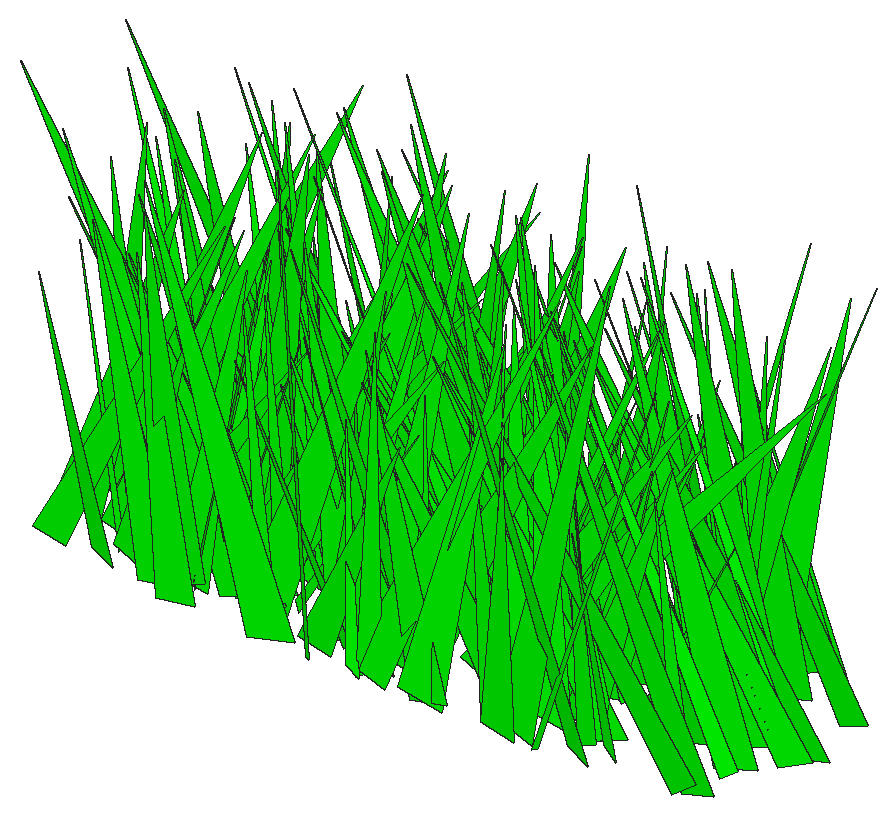
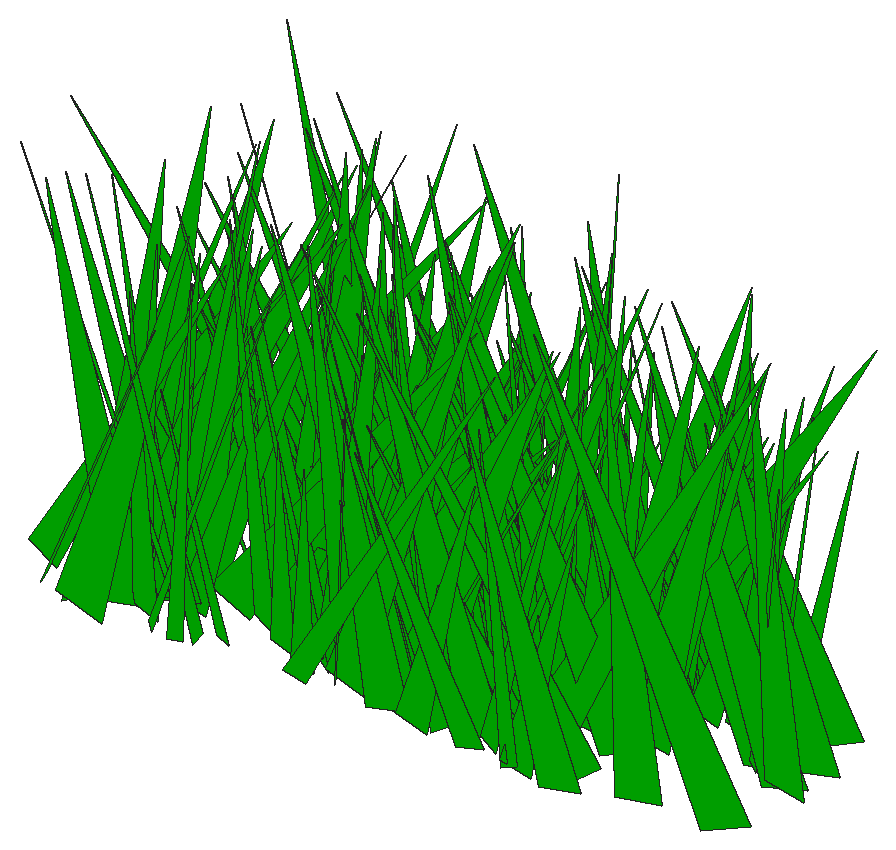
# SketchUp Ruby script. Lengths in inches.
U = 1.inch
M = Sketchup.active_model
def pt(a) = Geom::Point3d.new(a.map { |v| v * U })
def face(e, loops, mat)
  f = e.add_face(loops[0].map { |a| pt(a) })
  loops[1..].each { |l| e.add_face(l.map { |a| pt(a) }).erase! }
  f.material = f.back_material = mat if mat
  f
end
# faces: each face lists its corners as indices into pts; further lists are holes
def faces(e, pts, list, mat = nil) = list.each { |f| face(e, (f[0].is_a?(Array) ? f : [f]).map { |l| l.map { |i| pts[i] } }, mat) }
# xy, xz, yz: faces in a plane at the given z, y or x. An outline is a flat list of corners, or four numbers for a rectangle; further outlines are holes
def ring(l) = l.size == 4 ? [[l[0], l[1]], [l[2], l[1]], [l[2], l[3]], [l[0], l[3]]] : l.each_slice(2).to_a
def flat(e, list, mat, &to3) = list.each { |f| face(e, (f[0].is_a?(Array) ? f : [f]).map { |l| ring(l).map { |u, v| to3.(u, v) } }, mat) }
def xy(e, z, list, mat = nil) = flat(e, list, mat) { |x, y| [x, y, z] }
def xz(e, y, list, mat = nil) = flat(e, list, mat) { |x, z| [x, y, z] }
def yz(e, x, list, mat = nil) = flat(e, list, mat) { |y, z| [x, y, z] }
def lines(e, pts, list) = list.each { |a, b| e.add_line(pt(pts[a]), pt(pts[b])) }
# prism: a flat outline (further loops are holes) pulled along v
def prism(e, loops, v, mat = nil)
  f = face(e, loops, mat); d = Geom::Vector3d.new(v.map { |x| x * U })
  f.pushpull(f.normal.samedirection?(d) ? d.length : -d.length)
end
def box(e, o, s, mat = nil) = prism(e, [[o, [o[0] + s[0], o[1], o[2]], [o[0] + s[0], o[1] + s[1], o[2]], [o[0], o[1] + s[1], o[2]]]], [0, 0, s[2]], mat)
def at(x, y, z, deg = 0) = Geom::Transformation.translation(pt([x, y, z])) * Geom::Transformation.rotation(ORIGIN, Z_AXIS, deg.degrees)
def axes(o, x, y, z) = Geom::Transformation.new([*x, 0, *y, 0, *z, 0, *pt(o).to_a, 1])
def part(name) = M.definitions.add(name)
# library, detail: a bought-in or finely detailed component or shape, given as its bounding box
def library(name, o, s) = part(name).tap { |d| box(d.entities, o, s) }
def detail(e, o, s) = box(e.add_group.entities, o, s)
def put(e, d, t, mat = nil) = e.add_instance(d, t).tap { |i| i.material = mat if mat }
def group(e, t, mat = nil) = e.add_group.tap { |g| g.transformation = t; g.material = mat if mat }.entities
root = M.entities
M.materials.add("[0065_Lime]").color = [0, 255, 0]
c1 = part("fur_instance\#9")
p = [[0.8125,0,1.79],[0.67,-0.02,1.48],[0,-0.11,0],[0,0.11,0]]
faces(c1.entities,p,[[0,1,2,3]])
put(root,c1,axes([108.88,22.01,1.48],[4.75681,0.31747,1.98714],[-1.73779,0.74773,-1.25061],[-2.83772,0.07427,4.09688]),"[0065_Lime]")
put(root,c1,axes([107.32,22.59,1.48],[6.25624,-0.79402,0.40121],[5.39104,0.86446,1.70714],[-1.76366,-0.17423,6.64148]),"[0065_Lime]")
put(root,c1,axes([109.46,19.48,1.48],[-4.41361,-0.5637,0.07811],[3.85361,-0.60101,-1.27006],[1.11893,-0.15362,4.68226]),"[0065_Lime]")
put(root,c1,axes([109.5,20.23,1.48],[-5.51832,-0.04616,1.49049],[-0.04816,-0.8017,-0.94997],[1.86099,-0.15763,4.39513]),"[0065_Lime]")
put(root,c1,axes([107.19,21.34,1.48],[0.70179,-0.92138,2.00617],[6.79563,0.00491,-1.49729],[1.70207,0.36029,5.15083]),"[0065_Lime]")
put(root,c1,axes([109.98,20.83,1.48],[1.44553,0.98915,0.74754],[-6.89592,0.22695,-1.23991],[-1.68599,-0.08018,5.71232]),"[0065_Lime]")
put(root,c1,axes([110.23,20.91,1.48],[-6.41375,-0.00562,1.37592],[-0.3444,-0.90798,-1.18641],[1.65658,-0.21051,5.08044]),"[0065_Lime]")
put(root,c1,axes([111.48,20.82,1.48],[-6.87392,0.44824,1.7955],[-3.78696,-0.91218,-1.96188],[0.84068,-0.44398,5.8435]),"[0065_Lime]")
put(root,c1,axes([111.86,22.17,1.48],[-7.88942,0.4529,0.7145],[-3.09052,-1.10969,0.99166],[1.2683,0.11323,6.86094]),"[0065_Lime]")
put(root,c1,axes([114.3,20.58,1.48],[-2.0795,-1.15537,3.24941],[8.27079,0.00739,3.59006],[-3.89334,0.6328,5.89095]),"[0065_Lime]")
put(root,c1,axes([107.39,22.47,1.48],[5.1427,-0.91278,1.2703],[6.65541,0.67577,-1.556],[0.58303,0.33719,6.55712]),"[0065_Lime]")
put(root,c1,axes([111.92,22.77,1.48],[-1.07651,1.07847,0.62911],[-7.57075,-0.12668,-1.29461],[-1.47884,-0.13655,6.16966]),"[0065_Lime]")
put(root,c1,axes([111.49,19.3,1.48],[0.79576,0.87208,1.47847],[-6.2297,0.17243,-1.18969],[-1.73544,-0.2191,4.94855]),"[0065_Lime]")
put(root,c1,axes([107.26,25.14,1.48],[-2.18706,1.12852,2.58398],[-7.41501,-0.48145,2.89338],[4.42819,-0.24882,6.12118]),"[0065_Lime]")
put(root,c1,axes([113.59,20.85,1.48],[-5.58166,-0.54943,0.1697],[3.77911,-0.74255,1.68284],[-1.02475,0.25424,5.28174]),"[0065_Lime]")
put(root,c1,axes([107.625,19.53,1.48],[6.43557,-0.59106,0.78827],[4.3016,0.85789,-1.68113],[0.35835,0.31678,6.02355]),"[0065_Lime]")
put(root,c1,axes([114.28,23.85,1.48],[-6.00567,-0.99,0.85658],[6.98711,-0.78092,2.16878],[-1.38798,0.35246,7.21128]),"[0065_Lime]")
put(root,c1,axes([108.49,21.82,1.48],[8.65109,-0.17974,0.61801],[0.66489,1.03061,3.88566],[-1.3309,-0.65345,5.95838]),"[0065_Lime]")
put(root,c1,axes([109.99,25.4375,1.48],[-2.32113,-1.09259,0.4435],[7.51688,-0.33492,-1.61844],[2.06205,-0.00898,6.39898]),"[0065_Lime]")
put(root,c1,axes([108.86,20.88,1.48],[4.52414,0.72389,0.76271],[-5.23046,0.61658,0.9183],[0.24588,-0.2033,5.50075]),"[0065_Lime]")
put(root,c1,axes([112.42,20.94,1.48],[-6.35456,0.66956,0.55453],[-4.63808,-0.89415,1.01161],[1.28754,0.08357,6.38094]),"[0065_Lime]")
put(root,c1,axes([112.68,21.36,1.48],[4.49242,0.96826,0.54109],[-5.75128,0.58404,-3.42722],[-3.85307,0.25715,5.74652]),"[0065_Lime]")
put(root,c1,axes([109.91,19.96,1.48],[-2.07932,-0.66053,1.31721],[4.38724,-0.3598,-1.46364],[2.33894,0.08769,3.91639]),"[0065_Lime]")
put(root,c1,axes([108.47,21.99,1.48],[5.47429,0.98354,0.81524],[-7.02248,0.73547,1.46742],[0.82545,-0.26578,7.07742]),"[0065_Lime]")
put(root,c1,axes([112.79,23.15,1.48],[0.36017,-1.13824,1.08313],[8.05483,0.08514,1.22574],[-1.58371,0.17414,6.48052]),"[0065_Lime]")
put(root,c1,axes([113.59,20.08,1.48],[-0.45294,0.79492,1.39232],[-5.53302,0.02778,-1.72246],[-2.07798,-0.24725,4.28287]),"[0065_Lime]")
put(root,c1,axes([112.48,18.79,1.48],[1.21549,0.89008,0.72447],[-6.21056,0.19472,-1.12208],[-1.53157,-0.08319,5.12502]),"[0065_Lime]")
put(root,c1,axes([112.08,19.625,1.48],[4.98292,-0.96258,0.19503],[6.39598,0.66793,2.34476],[-2.46469,-0.21275,6.47907]),"[0065_Lime]")
put(root,c1,axes([114.55,20.11,1.48],[-2.22166,0.79723,0.80505],[-5.49656,-0.24901,-1.77319],[-1.71947,-0.23408,4.62809]),"[0065_Lime]")
put(root,c1,axes([114,22.82,1.48],[-2.51218,0.56119,0.72618],[-4.00317,-0.30645,-1.2272],[-0.84932,-0.21549,3.63629]),"[0065_Lime]")
put(root,c1,axes([114.17,20.66,1.48],[-2.35921,-1.01795,0.20784],[7.1664,-0.32186,0.99863],[-1.08993,0.08714,6.11622]),"[0065_Lime]")
put(root,c1,axes([111.86,21.4,1.48],[-5.14477,0.60785,0.71079],[-3.35714,-0.66147,2.87761],[2.86458,0.3165,4.64899]),"[0065_Lime]")
put(root,c1,axes([113.64,22.29,1.48],[-6.77708,0.59996,0.57809],[-3.92781,-0.93039,1.88959],[1.81862,0.22633,6.23535]),"[0065_Lime]")
put(root,c1,axes([111.94,23.04,1.48],[4.32561,0.38631,0.37978],[-2.5286,0.59443,-1.20585],[-1.17567,0.14285,3.9908]),"[0065_Lime]")
put(root,c1,axes([114.08,20.16,1.48],[-0.38061,-0.81633,1.21559],[5.84728,-0.00353,1.13197],[-1.3388,0.21667,4.59834]),"[0065_Lime]")
put(root,c1,axes([110.14,20.54,1.48],[3.92345,-0.53628,0.94206],[3.819,0.43935,-2.14273],[1.14972,0.37068,3.90264]),"[0065_Lime]")
put(root,c1,axes([113.64,26.11,1.48],[1.01933,-0.67584,0.27572],[4.63432,0.15077,1.0475],[-1.33061,0.00736,3.85949]),"[0065_Lime]")
put(root,c1,axes([112.12,19.8,1.48],[2.95244,-0.66107,2.58793],[5.66677,0.3764,-1.05566],[-0.37755,0.47991,4.39281]),"[0065_Lime]")
put(root,c1,axes([113.6,23.21,1.48],[6.49926,-0.57584,2.86664],[4.03045,1.03237,0.90299],[-3.60122,0.11618,6.18415]),"[0065_Lime]")
put(root,c1,axes([112.33,19.8125,1.48],[6.78722,0.16059,1.38807],[-0.6006,0.94692,-1.72789],[-1.96403,0.26539,5.32521]),"[0065_Lime]")
put(root,c1,axes([115.75,18.77,1.48],[-4.23697,0.9376,1.31798],[-6.84398,-0.55507,-1.32537],[-0.5542,-0.31336,6.29115]),"[0065_Lime]")
put(root,c1,axes([116.09,23.7,1.48],[-9.10693,-0.06064,1.00007],[0.17761,-1.26614,-1.5026],[1.29085,-0.25362,7.26219]),"[0065_Lime]")
put(root,c1,axes([115.02,25.53,1.48],[-5.8261,-0.37077,1.50453],[3.04674,-0.8087,1.12797],[1.04928,0.28945,5.07865]),"[0065_Lime]")
put(root,c1,axes([111.99,26.27,1.48],[1.22642,-0.90787,0.30312],[6.29841,0.15519,-1.28521],[1.48734,0.09141,5.19254]),"[0065_Lime]")
put(root,c1,axes([112.79,20.4,1.48],[5.14158,0.13277,0.67971],[-0.67571,0.70606,-1.23959],[-1.0651,0.19299,4.06757]),"[0065_Lime]")
put(root,c1,axes([112.34,21.03,1.48],[-2.53483,0.95653,2.95117],[-7.12293,-0.49622,1.34139],[2.96051,-0.3749,5.75419]),"[0065_Lime]")
put(root,c1,axes([112.46,22.05,1.48],[0.56511,0.56516,0.38968],[-3.7117,0.04505,1.37222],[1.62152,-0.09385,3.00523]),"[0065_Lime]")
put(root,c1,axes([113.23,21.25,1.48],[0.21192,-1.1921,1.83278],[8.70845,-0.01117,-0.90969],[1.10098,0.31781,6.84266]),"[0065_Lime]")
put(root,c1,axes([114.74,23.37,1.48],[-4.45858,-0.65966,0.8551],[4.54422,-0.6436,-0.96036],[1.5791,-0.01043,5.17802]),"[0065_Lime]")
put(root,c1,axes([114.6,20.02,1.48],[-5.51128,0.12231,2.48203],[-2.12772,-0.77996,-1.83809],[2.35399,-0.41864,4.14963]),"[0065_Lime]")
put(root,c1,axes([115.2,22.08,1.48],[-7.4027,0.42566,2.73576],[-3.72336,-1.0878,-0.99465],[2.57381,-0.3494,6.4296]),"[0065_Lime]")
put(root,c1,axes([113.82,26.14,1.48],[5.24176,0.29944,2.16883],[-3.01127,0.72897,1.44279],[-1.60707,-0.38923,4.3706]),"[0065_Lime]")
put(root,c1,axes([117.45,23.07,1.48],[-6.65793,-0.86672,0.90402],[6.2657,-0.91523,1.12903],[-0.14464,0.24903,7.29565]),"[0065_Lime]")
put(root,c1,axes([111.94,23.67,1.48],[-3.03044,1.05577,2.21873],[-6.67995,-0.55962,2.88653],[4.38979,-0.12274,5.9241]),"[0065_Lime]")
put(root,c1,axes([115.4375,22.41,1.48],[1.84297,1.05998,1.58754],[-7.62241,0.30371,-0.94025],[-1.61588,-0.2237,6.24601]),"[0065_Lime]")
put(root,c1,axes([114.8125,20.5,1.48],[5.76147,-0.43307,1.32614],[2.30483,0.80508,2.18459],[-2.61617,-0.24446,4.84511]),"[0065_Lime]")
put(root,c1,axes([118.36,24.63,1.48],[-8.66441,0.10283,0.01318],[-0.72259,-1.20595,0.97318],[0.11668,0.16733,7.00557]),"[0065_Lime]")
put(root,c1,axes([116.27,23.9,1.48],[1.54175,0.61801,1.12889],[-4.15611,0.27531,-1.29491],[-1.99901,-0.09575,3.56289]),"[0065_Lime]")
put(root,c1,axes([114.83,22.57,1.48],[-2.20909,0.81477,0.06052],[-5.52498,-0.29913,1.51072],[1.76097,0.0836,4.81576]),"[0065_Lime]")
put(root,c1,axes([117.61,19.7,1.48],[-4.71309,-0.23078,0.31888],[1.6872,-0.63733,1.04366],[-0.06575,0.18829,3.92334]),"[0065_Lime]")
put(root,c1,axes([114.79,23.65,1.48],[-6.53595,-0.6054,2.38454],[3.40148,-0.99622,-2.30654],[3.94784,-0.14393,5.9351]),"[0065_Lime]")
put(root,c1,axes([113.04,20.89,1.48],[3.67559,-0.76857,0.24402],[5.32315,0.48917,-1.42317],[1.29237,0.171,5.16789]),"[0065_Lime]")
put(root,c1,axes([118.3125,24.52,1.48],[-2.28678,1.15619,0.4981],[-8.03755,-0.29199,-1.70332],[-1.86378,-0.15937,6.73442]),"[0065_Lime]")
put(root,c1,axes([111.93,25.12,1.48],[7.61782,-0.42793,0.14657],[2.94088,1.01199,-2.12453],[0.81116,0.34978,6.32601]),"[0065_Lime]")
put(root,c1,axes([111.79,22.7,1.48],[5.17986,-0.77049,0.06287],[5.04502,0.6637,-2.45936],[2.14937,0.299,5.62112]),"[0065_Lime]")
put(root,c1,axes([116.96,20.71,1.48],[-0.18332,-0.59721,0.87484],[4.22584,0.0162,0.95637],[-1.16707,0.15245,3.32548]),"[0065_Lime]")
put(root,c1,axes([117.81,20.99,1.48],[-7.05017,0.06409,0.7695],[-0.25595,-0.97987,1.18316],[1.01855,0.19739,5.62357]),"[0065_Lime]")
put(root,c1,axes([114.29,24.84,1.48],[-1.69328,-1.27873,0.40691],[8.7177,-0.2481,-2.12324],[2.65778,-0.00089,7.22362]),"[0065_Lime]")
put(root,c1,axes([117.32,25.92,1.48],[0.67945,0.70964,1.24411],[-5.01954,0.15375,-1.12489],[-1.62727,-0.17795,3.98934]),"[0065_Lime]")
put(root,c1,axes([115.96,24.12,1.48],[3.20358,0.43841,0.0671],[-2.92117,0.42703,-1.21601],[-1.09889,0.1429,3.42813]),"[0065_Lime]")
put(root,c1,axes([116.34,21.95,1.48],[-4.33322,-0.2806,1.31295],[1.69913,-0.64693,-0.92263],[1.92507,-0.06061,3.76969]),"[0065_Lime]")
put(root,c1,axes([117.49,20,1.48],[1.80855,1.06223,0.18183],[-7.2575,0.25285,-1.73635],[-2.12693,0.04045,6.07937]),"[0065_Lime]")
put(root,c1,axes([114.125,21.95,1.48],[-0.07185,1.2934,0.07562],[-8.85908,-0.01326,2.03283],[2.49988,-0.00983,7.2061]),"[0065_Lime]")
put(root,c1,axes([117.12,18.61,1.48],[7.88751,0.15029,3.42144],[-0.47652,1.24861,-1.11101],[-4.31389,0.13687,6.37848]),"[0065_Lime]")
put(root,c1,axes([120.32,24.45,1.48],[-4.53183,1.05701,0.11134],[-7.24742,-0.60731,-1.98181],[-2.01934,-0.19252,6.86289]),"[0065_Lime]")
put(root,c1,axes([119.54,22.58,1.48],[-7.74639,-0.18987,0.54799],[1.44778,-1.07452,1.06543],[0.42849,0.19802,6.3068]),"[0065_Lime]")
put(root,c1,axes([120.15,22.93,1.48],[-7.37445,0.23979,0.33216],[-1.70896,-0.92533,-2.71939],[-0.39788,-0.46995,5.52389]),"[0065_Lime]")
put(root,c1,axes([119.01,20.19,1.48],[-2.08243,0.70172,0.46791],[-4.84715,-0.25712,-1.35203],[-1.33208,-0.1614,4.18826]),"[0065_Lime]")
put(root,c1,axes([114.24,24.77,1.48],[3.79805,0.57077,0.31827],[-3.85368,0.47697,1.76436],[1.34222,-0.24566,4.16509]),"[0065_Lime]")
put(root,c1,axes([113.89,20.45,1.48],[3.51071,0.78023,0.49381],[-5.25387,0.42706,2.10303],[1.89635,-0.26126,4.91232]),"[0065_Lime]")
put(root,c1,axes([114.44,20.07,1.48],[6.76565,-0.83708,2.01476],[6.4503,0.88762,-1.97384],[-0.12735,0.48692,7.06186]),"[0065_Lime]")
put(root,c1,axes([115.89,23.16,1.48],[-3.1916,-0.77323,2.59515],[5.69373,-0.5709,-1.06685],[2.83556,0.27603,5.0632]),"[0065_Lime]")
put(root,c1,axes([115.28,25.98,1.48],[2.3863,0.6485,0.60605],[-4.56285,0.29752,1.21908],[1.01725,-0.18676,4.04648]),"[0065_Lime]")
put(root,c1,axes([114.39,22.34,1.48],[5.26977,-0.54033,0.30957],[3.79475,0.70663,-1.41195],[0.72856,0.22776,5.11503]),"[0065_Lime]")
put(root,c1,axes([115.15,20.64,1.48],[4.78228,0.13087,0.01494],[-0.89815,0.64419,1.12549],[0.24722,-0.19132,3.79988]),"[0065_Lime]")
put(root,c1,axes([115.42,25.35,1.48],[0.23421,-1.08101,2.16362],[7.81278,-0.07509,-1.81665],[2.28442,0.36762,5.99115]),"[0065_Lime]")
put(root,c1,axes([120.08,25.29,1.48],[4.54453,0.80887,4.60833],[-6.54285,0.90426,-1.04944],[-4.73539,-0.47314,5.87259]),"[0065_Lime]")
put(root,c1,axes([118.91,21.45,1.48],[-4.66798,0.18091,0.42592],[-1.08616,-0.6357,1.17185],[0.8672,0.17761,3.7604]),"[0065_Lime]")
put(root,c1,axes([116.48,25.56,1.48],[-5.97897,-0.8659,1.63522],[4.93662,-0.85736,-3.27031],[4.20046,-0.22491,6.17104]),"[0065_Lime]")
put(root,c1,axes([116.89,24.8,1.48],[-0.93274,0.72478,1.44432],[-5.25377,-0.18747,0.90751],[1.46789,-0.21044,4.16585]),"[0065_Lime]")
put(root,c1,axes([116.77,20.32,1.48],[-5.33037,0.70186,1.45724],[-3.84774,-0.75694,2.9042],[3.65413,0.22677,5.18378]),"[0065_Lime]")
put(root,c1,axes([119.18,19.52,1.48],[-5.78186,-0.32004,0.6774],[2.09686,-0.81176,-1.00964],[1.21821,-0.12171,4.95292]),"[0065_Lime]")
put(root,c1,axes([116.67,20.41,1.48],[7.33665,-0.52864,0.50322],[3.29109,0.97329,2.51445],[-1.9248,-0.35083,6.21738]),"[0065_Lime]")
put(root,c1,axes([121.33,25.88,1.48],[-7.42153,0.39429,0.17707],[-2.78536,-1.01665,-1.38433],[-0.40322,-0.23434,6.30361]),"[0065_Lime]")
put(root,c1,axes([120.53,19.48,1.48],[-6.78605,-0.44371,1.28341],[3.51607,-0.8922,1.96457],[0.31266,0.40299,5.76251]),"[0065_Lime]")
put(root,c1,axes([118.51,18.78,1.48],[-4.45554,0.29398,0.76074],[-1.6058,-0.6055,1.61806],[1.63496,0.20645,3.66233]),"[0065_Lime]")
put(root,c1,axes([116.86,19.22,1.48],[0.87841,-0.73867,0.02479],[5.04663,0.11728,-1.21777],[1.47184,0.03873,4.16068]),"[0065_Lime]")
put(root,c1,axes([122.1875,22.21,1.48],[-3.38223,-0.67748,0.64954],[4.32175,-0.35094,2.62408],[-2.28146,0.33957,4.00785]),"[0065_Lime]")
put(root,c1,axes([119.83,23.92,1.48],[-5.47386,-0.14391,1.0743],[0.66616,-0.77074,-1.21387],[1.53278,-0.17896,4.36409]),"[0065_Lime]")
put(root,c1,axes([117.8,20.84,1.48],[6.55865,-0.63822,2.86701],[5.55432,0.89734,-1.7134],[-1.48379,0.538,6.25893]),"[0065_Lime]")
put(root,c1,axes([120.92,22.9,1.48],[-3.03016,-1.18286,2.10117],[8.78455,-0.37977,1.2181],[-0.60401,0.41089,7.17464]),"[0065_Lime]")
put(root,c1,axes([121.56,22.23,1.48],[-0.58168,1.07553,3.09864],[-8.21284,0.07882,-1.93679],[-2.37608,-0.53573,5.93589]),"[0065_Lime]")
put(root,c1,axes([118.27,25.61,1.48],[5.00089,-0.23631,0.58981],[1.43452,0.68964,1.21137],[-1.13849,-0.16906,4.11713]),"[0065_Lime]")
put(root,c1,axes([118.9,19,1.48],[6.15038,-0.52199,1.19737],[3.22978,0.87297,1.77594],[-2.35269,-0.16618,5.56817]),"[0065_Lime]")
put(root,c1,axes([119.15,21.14,1.48],[5.05279,-0.24169,1.22034],[1.01446,0.69657,1.84367],[-2.04453,-0.25168,3.9307]),"[0065_Lime]")
put(root,c1,axes([121.82,21.36,1.48],[-5.27601,0.45464,0.36816],[-3.25893,-0.72395,-0.94344],[-0.22895,-0.17197,4.94507]),"[0065_Lime]")
put(root,c1,axes([117.53,25.19,1.48],[7.65657,0.04562,1.09105],[-0.73546,1.03397,1.96609],[-1.16776,-0.35207,5.91538]),"[0065_Lime]")
put(root,c1,axes([118.28,25.73,1.48],[-0.86023,-0.99421,0.49878],[6.80499,-0.14022,-1.60067],[2.0318,0.04871,5.57219]),"[0065_Lime]")
put(root,c1,axes([121.11,18.75,1.48],[1.35591,0.83981,1.29808],[-5.86256,0.24771,-1.31835],[-1.97382,-0.15883,4.80744]),"[0065_Lime]")
put(root,c1,axes([123.15,22.43,1.48],[-1.84543,-1.23425,1.90817],[8.65227,-0.13516,2.60709],[-2.79147,0.39704,6.81928]),"[0065_Lime]")
put(root,c1,axes([120.51,25.13,1.48],[-5.85625,0.07812,1.72253],[0.41265,-0.79512,2.13666],[2.15018,0.36538,4.28143]),"[0065_Lime]")
put(root,c1,axes([123.71,21.6,1.48],[-4.77751,0.58364,0.27694],[-3.75387,-0.57107,-2.5182],[-1.81001,-0.35615,4.49164]),"[0065_Lime]")
put(root,c1,axes([120.8125,24.79,1.48],[5.51324,-0.87776,0.99225],[5.64963,0.77936,2.33265],[-2.93089,-0.14883,6.36296]),"[0065_Lime]")
put(root,c1,axes([119.12,23.35,1.48],[0.62244,0.70849,0.87955],[-5.00092,0.04561,1.11055],[1.25776,-0.16928,3.98036]),"[0065_Lime]")
put(root,c1,axes([120.24,24.79,1.48],[6.49909,0.95529,0.52041],[-6.29431,0.88622,-2.50314],[-2.64731,0.23809,7.22911]),"[0065_Lime]")
put(root,c1,axes([121.32,22.29,1.48],[1.02109,-1.08574,0.0472],[7.64617,0.14316,0.90803],[-1.11425,-0.01255,6.27429]),"[0065_Lime]")
put(root,c1,axes([120.9375,23.125,1.48],[2.50794,0.80047,0.27755],[-5.56145,0.35456,-1.01625],[-1.27987,0.02786,4.95983]),"[0065_Lime]")
put(root,c1,axes([120.93,21.49,1.48],[-6.29754,0.28767,1.72302],[-0.88384,-0.85463,2.64386],[2.81013,0.37586,4.69286]),"[0065_Lime]")
put(root,c1,axes([123.21,19.71,1.48],[0.92262,-0.87538,0.67989],[5.52158,0.1696,2.35948],[-3.00327,0.04289,4.54682]),"[0065_Lime]")
put(root,c1,axes([118.5,24.87,1.48],[1.78241,-1.15471,0.51368],[8.00538,0.22097,-1.73401],[1.9597,0.14756,6.61622]),"[0065_Lime]")
put(root,c1,axes([117.92,21.88,1.48],[5.81279,0.63106,0.00545],[-4.41707,0.80308,1.08633],[0.8113,-0.14907,5.87539]),"[0065_Lime]")
put(root,c1,axes([120.27,21.86,1.48],[-4.69664,-0.91781,1.37829],[6.05408,-0.70126,-1.99813],[2.98014,-0.02186,6.2313]),"[0065_Lime]")
put(root,c1,axes([121.29,25.59,1.48],[-2.93693,0.50067,0.15322],[-3.41179,-0.40411,0.9779],[1.04414,0.08782,3.62633]),"[0065_Lime]")
put(root,c1,axes([125.1875,23.78,1.48],[-5.44815,0.81973,0.96618],[-5.55931,-0.61958,-3.1268],[-2.12979,-0.47965,5.69021]),"[0065_Lime]")
put(root,c1,axes([118.2,21.76,1.48],[7.16849,0.77844,1.90301],[-6.01271,0.91912,2.38724],[0.10214,-0.5272,6.97184]),"[0065_Lime]")
put(root,c1,axes([122.95,22.78,1.48],[-1.41699,0.72489,0.97846],[-5.13613,-0.14521,-1.3164],[-1.29585,-0.21709,4.14767]),"[0065_Lime]")
put(root,c1,axes([125.2,22.29,1.48],[-5.42074,0.38654,0.03939],[-2.52569,-0.69319,-2.03181],[-1.09104,-0.31582,4.50782]),"[0065_Lime]")
put(root,c1,axes([118.91,18.86,1.48],[6.33349,0.90822,0.60373],[-6.47232,0.86483,1.329],[0.65996,-0.23449,7.23979]),"[0065_Lime]")
put(root,c1,axes([120.85,18.72,1.48],[-2.78902,0.94375,1.61298],[-6.48391,-0.46132,1.6268],[2.64564,-0.1357,5.68732]),"[0065_Lime]")
put(root,c1,axes([121.3,24.77,1.48],[5.85912,0.47031,0.62649],[-3.00871,0.80608,-1.65999],[-1.65629,0.19945,5.23164]),"[0065_Lime]")
put(root,c1,axes([122.55,24.83,1.48],[2.14179,0.565,0.18937],[-3.86834,0.29889,-0.93463],[-1.12136,0.04807,3.58588]),"[0065_Lime]")
put(root,c1,axes([122.97,19.17,1.48],[3.0262,0.58862,1.21834],[-3.98394,0.47185,-1.09153],[-1.97955,-0.04979,4.05926]),"[0065_Lime]")
put(root,c1,axes([123.125,20.11,1.48],[-4.86138,0.82668,0.80414],[-5.69414,-0.69645,1.21537],[1.77897,0.02984,6.08763]),"[0065_Lime]")
put(root,c1,axes([122.45,21.97,1.48],[-3.25218,0.61462,0.68324],[-4.03718,-0.46852,1.4083],[1.88101,0.05706,4.2039]),"[0065_Lime]")
put(root,c1,axes([119.74,19.71,1.48],[4.44404,-0.97779,0.88545],[6.88012,0.564,-1.97731],[1.5065,0.30865,6.41829]),"[0065_Lime]")
put(root,c1,axes([124.98,23.11,1.48],[-0.84639,-0.78047,0.35779],[5.25673,-0.09114,1.56576],[-1.84652,0.09828,4.29344]),"[0065_Lime]")
put(root,c1,axes([126.1875,20.18,1.48],[-4.81737,0.65495,0.08588],[-4.48491,-0.64519,-1.57446],[-1.27345,-0.20537,5.22014]),"[0065_Lime]")
put(root,c1,axes([124.21,21.76,1.48],[2.5245,-1.16462,2.00194],[8.34624,0.42229,1.26832],[-2.25603,0.25906,6.93236]),"[0065_Lime]")
put(root,c1,axes([124.59,21.47,1.48],[-0.53859,-0.67612,1.08932],[4.83092,-0.02248,1.11288],[-1.26782,0.20158,3.77777]),"[0065_Lime]")
put(root,c1,axes([123.32,18.78,1.48],[5.75086,-0.0612,2.22428],[1.02934,0.8695,-0.95913],[-2.57054,0.21125,4.59213]),"[0065_Lime]")
put(root,c1,axes([123.98,20.78,1.48],[1.763,1.2588,0.5016],[-8.86984,0.25789,-1.05969],[-1.39903,-0.04872,7.35057]),"[0065_Lime]")
put(root,c1,axes([124.4,19.89,1.48],[-6.61511,0.78758,1.06019],[-5.2713,-0.94129,1.66953],[2.3079,0.10749,6.85206]),"[0065_Lime]")
put(root,c1,axes([124.35,22.34,1.48],[-5.26008,-0.66555,0.88682],[4.49548,-0.75204,-1.27006],[1.84736,-0.06498,5.61573]),"[0065_Lime]")
put(root,c1,axes([123.56,18.64,1.48],[-2.17411,-0.77393,0.45117],[5.37048,-0.3152,-0.99478],[1.3418,0.00756,4.7126]),"[0065_Lime]")
put(root,c1,axes([126.03,18.94,1.48],[-7.84081,-0.57692,0.60724],[3.98426,-1.10136,-1.02432],[1.24086,-0.10915,7.12604]),"[0065_Lime]")
put(root,c1,axes([123.84,20.88,1.48],[3.80412,-0.76834,0.94512],[5.35806,0.55747,0.91721],[-1.5936,0.04023,5.33999]),"[0065_Lime]")
put(root,c1,axes([123.66,24.19,1.48],[6.50209,0.60345,1.58222],[-3.96802,0.95193,-1.37678],[-2.54579,0.05751,6.18701]),"[0065_Lime]")
put(root,c1,axes([121.64,21,1.48],[7.71526,-0.30906,1.16385],[2.54643,1.03253,-1.98111],[-0.63282,0.38684,6.21774]),"[0065_Lime]")
put(root,c1,axes([126.02,26.12,1.48],[-7.20346,-0.10404,0.90757],[0.32947,-0.96919,-1.99276],[1.29791,-0.3314,5.54293]),"[0065_Lime]")
put(root,c1,axes([122.93,23.43,1.48],[0.52275,-1.10636,0.36151],[7.74658,0.06032,-1.22514],[1.47634,0.07521,6.30048]),"[0065_Lime]")
put(root,c1,axes([129.35,19.3,1.48],[-7.90762,-0.68912,0.40866],[4.57594,-0.97638,3.41374],[-1.83409,0.53511,6.75514]),"[0065_Lime]")
put(root,c1,axes([126.375,23.33,1.48],[-3.3827,-0.75365,0.70833],[5.40364,-0.45149,0.97738],[-0.56972,0.19254,5.0644]),"[0065_Lime]")
put(root,c1,axes([122.53,20.1875,1.48],[6.57385,0.35352,0.17052],[-2.40111,0.90091,-1.34097],[-0.77984,0.20621,5.56622]),"[0065_Lime]")
put(root,c1,axes([121.87,22.3,1.48],[1.33016,0.79555,0.39395],[-5.16755,0.14029,2.05089],[2.36318,-0.14101,4.26292]),"[0065_Lime]")
put(root,c1,axes([125.98,20.18,1.48],[-7.88368,0.25258,2.16249],[-2.45442,-1.11291,-1.56458],[2.06751,-0.35806,6.38846]),"[0065_Lime]")
put(root,c1,axes([125.79,24.63,1.48],[0.88547,-0.61254,0.94064],[4.23482,0.16988,1.06933],[-1.55106,0.11414,3.45658]),"[0065_Lime]")
put(root,c1,axes([121.3,20.78,1.48],[0.71976,0.95657,2.30411],[-6.41741,-0.11566,2.93537],[3.63073,-0.39406,4.73157]),"[0065_Lime]")
put(root,c1,axes([125.05,20.82,1.48],[-4.64175,-0.16151,1.34391],[0.626,-0.6705,-1.26959],[1.91283,-0.1725,3.67666]),"[0065_Lime]")
put(root,c1,axes([125.05,26.29,1.48],[-5.63276,-0.47707,1.66741],[3.13849,-0.84209,-1.05852],[2.42458,-0.01829,5.24391]),"[0065_Lime]")
put(root,c1,axes([128.02,21.45,1.48],[-7.18007,-0.60784,1.01015],[4.50037,-0.97203,1.56528],[0.03144,0.32179,6.63629]),"[0065_Lime]")
put(root,c1,axes([125.85,19.55,1.48],[4.53735,0.54235,1.54029],[-3.32492,0.68793,-1.63642],[-2.7254,0.06367,4.56073]),"[0065_Lime]")
put(root,c1,axes([124.04,25.51,1.48],[4.43129,-0.21069,0.08724],[1.38066,0.589,1.26528],[-0.59451,-0.20255,3.5887]),"[0065_Lime]")
put(root,c1,axes([126.71,23.62,1.48],[0.44702,1.10892,0.87711],[-7.77761,0.0935,-1.33826],[-1.71747,-0.13477,6.28864]),"[0065_Lime]")
put(root,c1,axes([126.6875,24.61,1.48],[-8.12288,-0.63821,1.3691],[4.30906,-1.16304,-1.25175],[2.21209,-0.07797,7.46575]),"[0065_Lime]")
put(root,c1,axes([128.97,20.2,1.48],[-9.21029,-0.01216,0.15168],[0.11571,-1.27724,1.21711],[0.16992,0.21053,7.39258]),"[0065_Lime]")
put(root,c1,axes([122.25,21.18,1.48],[4.98881,0.62104,0.32485],[-4.25543,0.64556,1.88424],[1.25854,-0.27897,5.08336]),"[0065_Lime]")
put(root,c1,axes([123.46,22.11,1.48],[4.22288,0.48182,0.45964],[-3.46009,0.57134,0.96418],[0.32307,-0.17885,4.31837]),"[0065_Lime]")
put(root,c1,axes([123.85,18.94,1.48],[6.69073,0.82504,2.51266],[-6.53644,0.92533,1.33477],[-1.13633,-0.46485,7.11666]),"[0065_Lime]")
put(root,c1,axes([129.54,22.38,1.48],[-3.55515,1.07218,0.82066],[-7.29372,-0.41946,-2.54229],[-2.45768,-0.30613,6.3577]),"[0065_Lime]")
put(root,c1,axes([124.76,20.75,1.48],[-2.21156,-0.5713,2.12694],[4.23308,-0.42399,-0.9039],[2.33411,0.22763,3.65456]),"[0065_Lime]")
put(root,c1,axes([124.38,21.73,1.48],[7.2761,-0.43891,0.13724],[2.7927,0.93852,2.61278],[-1.40908,-0.4063,5.887]),"[0065_Lime]")
put(root,c1,axes([129.2,23.08,1.48],[-7.91409,-0.08171,0.22019],[0.62753,-1.08383,1.44556],[0.1328,0.25191,6.29083]),"[0065_Lime]")
put(root,c1,axes([124.41,22.32,1.48],[6.27245,-0.32929,1.29008],[2.69389,0.86077,-1.30384],[-0.86601,0.29256,5.28818]),"[0065_Lime]")
put(root,c1,axes([127.19,24.01,1.48],[-6.11803,0.70464,0.16803],[-4.73299,-0.82527,1.94622],[1.66953,0.24258,6.13312]),"[0065_Lime]")
put(root,c1,axes([127.79,22.46,1.48],[-5.97547,0.59924,0.24145],[-4.17004,-0.83287,0.98279],[0.94076,0.11441,5.88995]),"[0065_Lime]")
put(root,c1,axes([126.6,19.59,1.48],[-3.96121,-0.37697,0.34271],[2.34429,-0.52754,-1.51645],[1.37074,-0.18717,3.58388]),"[0065_Lime]")
put(root,c1,axes([124.59,25.88,1.48],[8.30226,-0.02352,1.52916],[0.52523,1.17339,-1.28195],[-1.81281,0.23224,6.63177]),"[0065_Lime]")
put(root,c1,axes([124.98,20.43,1.48],[2.20431,-0.76613,0.80054],[5.47502,0.27845,-1.04531],[0.84799,0.19374,4.66801]),"[0065_Lime]")
put(root,c1,axes([126.6,25.61,1.48],[4.26766,0.63527,1.21798],[-4.38767,0.63433,-0.91447],[-1.85181,-0.03894,4.97366]),"[0065_Lime]")
put(root,c1,axes([128.16,26.47,1.48],[3.67053,-1.03938,0.93398],[6.70963,0.53651,2.56024],[-3.31847,-0.06487,6.20964]),"[0065_Lime]")
put(root,c1,axes([127.93,24.52,1.48],[-0.13241,0.68278,0.30514],[-4.69839,-0.00387,-1.05839],[-1.29471,-0.05577,3.8096]),"[0065_Lime]")
put(root,c1,axes([124.91,18.52,1.48],[7.57751,0.27855,0.8484],[-1.76798,1.0612,-1.2272],[-1.37536,0.17051,6.25175]),"[0065_Lime]")
put(root,c1,axes([129.8,20.65,1.48],[-7.94767,0.25268,0.52666],[-1.88561,-1.10016,-1.13993],[0.31186,-0.21245,6.52939]),"[0065_Lime]")
put(root,c1,axes([127.5625,24.73,1.48],[-5.80695,0.52914,1.34941],[-3.5652,-0.8483,0.99531],[2.0546,0.02351,5.54097]),"[0065_Lime]")
put(root,c1,axes([121.84,21.94,1.48],[7.31163,0.79222,0.17365],[-5.05149,0.89737,3.5446],[2.5126,-0.50119,6.62099]),"[0065_Lime]")
put(root,c1,axes([129.83,19.3,1.48],[-5.61416,-0.72759,1.2989],[5.39588,-0.72115,1.8948],[-0.49556,0.3907,5.91635]),"[0065_Lime]")
put(root,c1,axes([128.61,26.33,1.48],[-5.42447,-0.42766,0.0822],[2.82299,-0.71712,-1.7603],[1.14167,-0.25872,4.74325]),"[0065_Lime]")
put(root,c1,axes([130.84,22.19,1.48],[-4.66842,0.72824,0.43868],[-4.93049,-0.5845,-2.20252],[-1.68521,-0.30731,5.22874]),"[0065_Lime]")
put(root,c1,axes([125.8,22.0625,1.48],[4.27418,0.06862,0.20971],[-0.54364,0.57255,1.05296],[-0.09706,-0.18497,3.33712]),"[0065_Lime]")
put(root,c1,axes([130.71,24.81,1.48],[-5.68155,-0.68961,0.73448],[4.90561,-0.73669,1.92995],[-0.91383,0.33281,5.79384]),"[0065_Lime]")
put(root,c1,axes([130.95,22.625,1.48],[-3.72933,-0.97916,0.01371],[6.68992,-0.50235,1.80579],[-1.9497,0.1492,6.16992]),"[0065_Lime]")
put(root,c1,axes([128.39,24.875,1.48],[3.67502,-1.07119,1.14817],[7.38064,0.55059,1.58236],[-2.3731,0.05354,6.69941]),"[0065_Lime]")
put(root,c1,axes([129.9,25.78,1.48],[-6.26256,0.06862,0.35049],[-0.36274,-0.8537,1.31208],[0.54087,0.22196,4.93817]),"[0065_Lime]")
put(root,c1,axes([129.75,21,1.48],[4.06205,-0.86032,3.34469],[6.24573,0.75208,1.46357],[-3.9222,0.30663,5.79454]),"[0065_Lime]")
put(root,c1,axes([128.08,20.72,1.48],[5.10441,-0.4027,0.97818],[1.97445,0.67111,2.44097],[-2.40013,-0.30434,4.08837]),"[0065_Lime]")
put(root,c1,axes([129.3,22.46,1.48],[1.30263,0.81773,0.74149],[-5.55983,0.21402,-1.44642],[-1.94549,-0.0641,4.63006]),"[0065_Lime]")
put(root,c1,axes([130.55,22.625,1.48],[-8.57694,0.08749,1.10129],[-0.94962,-1.17739,-1.75889],[1.14847,-0.32012,6.77021]),"[0065_Lime]")
put(root,c1,axes([129.33,22.84,1.48],[1.8999,-1.17827,1.86355],[8.41947,0.33139,1.34183],[-2.16184,0.25513,6.86362]),"[0065_Lime]")
put(root,c1,axes([126.23,24.6,1.48],[-1.74876,-0.9498,2.38375],[6.69656,-0.38136,-1.84137],[3.07119,0.29072,5.37232]),"[0065_Lime]")
put(root,c1,axes([126.03,24.95,1.48],[8.69915,0.21398,0.74847],[-1.20229,1.18262,-2.08393],[-1.31155,0.33519,6.87469]),"[0065_Lime]")
put(root,c1,axes([127.16,25.55,1.48],[-1.29194,1.02885,1.99898],[-7.4493,-0.25843,1.27153],[2.03882,-0.29227,5.91251]),"[0065_Lime]")
put(root,c1,axes([127.99,22.89,1.48],[6.48101,0.63968,0.84602],[-4.07568,0.89692,-2.06678],[-2.27912,0.21511,6.10175]),"[0065_Lime]")
